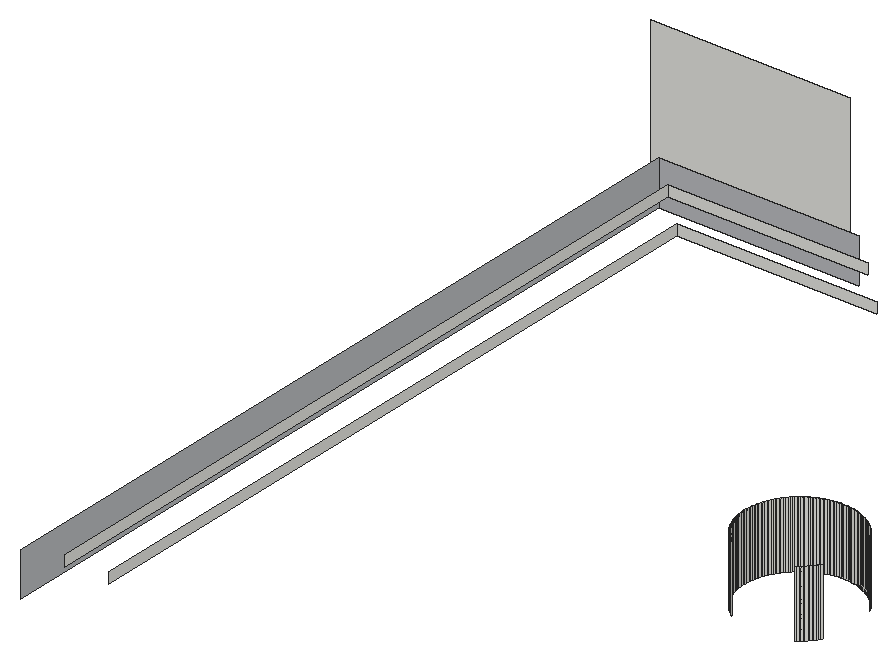
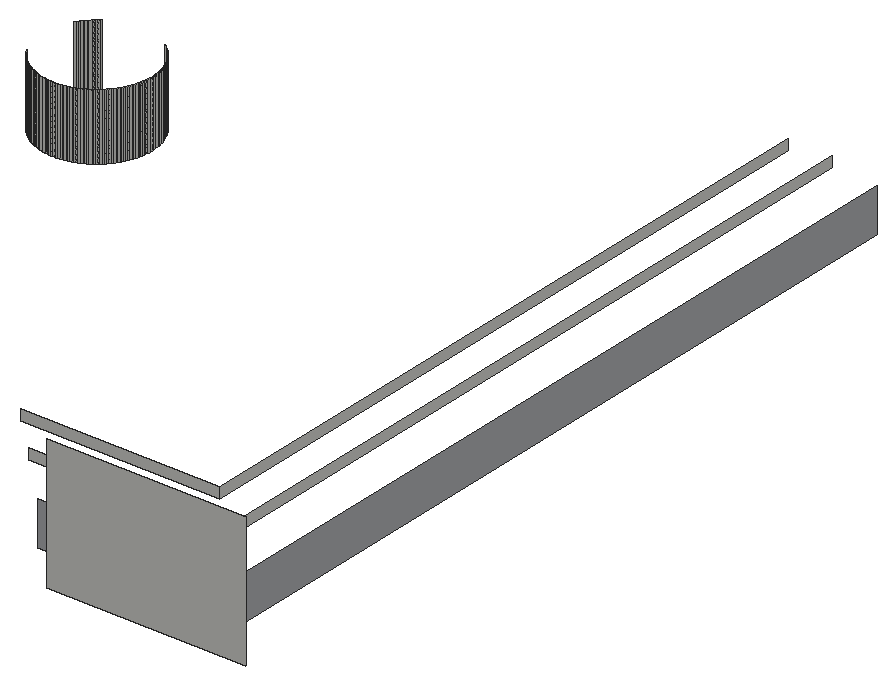
# SketchUp Ruby script. Lengths in inches.
U = 1.inch
M = Sketchup.active_model
def pt(a) = Geom::Point3d.new(a.map { |v| v * U })
def face(e, loops, mat)
  f = e.add_face(loops[0].map { |a| pt(a) })
  loops[1..].each { |l| e.add_face(l.map { |a| pt(a) }).erase! }
  f.material = f.back_material = mat if mat
  f
end
# faces: each face lists its corners as indices into pts; further lists are holes
def faces(e, pts, list, mat = nil) = list.each { |f| face(e, (f[0].is_a?(Array) ? f : [f]).map { |l| l.map { |i| pts[i] } }, mat) }
# xy, xz, yz: faces in a plane at the given z, y or x. An outline is a flat list of corners, or four numbers for a rectangle; further outlines are holes
def ring(l) = l.size == 4 ? [[l[0], l[1]], [l[2], l[1]], [l[2], l[3]], [l[0], l[3]]] : l.each_slice(2).to_a
def flat(e, list, mat, &to3) = list.each { |f| face(e, (f[0].is_a?(Array) ? f : [f]).map { |l| ring(l).map { |u, v| to3.(u, v) } }, mat) }
def xy(e, z, list, mat = nil) = flat(e, list, mat) { |x, y| [x, y, z] }
def xz(e, y, list, mat = nil) = flat(e, list, mat) { |x, z| [x, y, z] }
def yz(e, x, list, mat = nil) = flat(e, list, mat) { |y, z| [x, y, z] }
def lines(e, pts, list) = list.each { |a, b| e.add_line(pt(pts[a]), pt(pts[b])) }
# prism: a flat outline (further loops are holes) pulled along v
def prism(e, loops, v, mat = nil)
  f = face(e, loops, mat); d = Geom::Vector3d.new(v.map { |x| x * U })
  f.pushpull(f.normal.samedirection?(d) ? d.length : -d.length)
end
def box(e, o, s, mat = nil) = prism(e, [[o, [o[0] + s[0], o[1], o[2]], [o[0] + s[0], o[1] + s[1], o[2]], [o[0], o[1] + s[1], o[2]]]], [0, 0, s[2]], mat)
def at(x, y, z, deg = 0) = Geom::Transformation.translation(pt([x, y, z])) * Geom::Transformation.rotation(ORIGIN, Z_AXIS, deg.degrees)
def axes(o, x, y, z) = Geom::Transformation.new([*x, 0, *y, 0, *z, 0, *pt(o).to_a, 1])
def part(name) = M.definitions.add(name)
# library, detail: a bought-in or finely detailed component or shape, given as its bounding box
def library(name, o, s) = part(name).tap { |d| box(d.entities, o, s) }
def detail(e, o, s) = box(e.add_group.entities, o, s)
def put(e, d, t, mat = nil) = e.add_instance(d, t).tap { |i| i.material = mat if mat }
def group(e, t, mat = nil) = e.add_group.tap { |g| g.transformation = t; g.material = mat if mat }.entities
root = M.entities
M.materials.add("1427 AP 686 ARMOUR-N").color = [184, 186, 189]
xz(root,158.42,[[34.84,242,34.92,245],[34.92,242,35,245],[35,242,35.08,245],[35.08,242,35.16,245]])
xz(root,174,[[15,242,24,242.5]])
xz(root,176,[[13,242,22,242.5]])
xz(root,178,[[11,240,20,242]],"1427 AP 686 ARMOUR-N")
xz(root,180,[[9,240,18,246]])
yz(root,11,[[141.93,240,178,242]],"1427 AP 686 ARMOUR-N")
yz(root,13,[[141.9375,242,176,242.5]])
yz(root,15,[[141.94,242,174,242.5]])
yz(root,32.5,[[155.85,242,155.92,245],[155.92,242,156,245]])
yz(root,32.51,[[155.6875,242,155.77,245],[156.08,242,156.16,245]])
p = [[33.47,153.95,242],[33.41,154,242],[33.41,154,245],[33.47,153.95,245],[33.53,153.9,242],[33.53,153.9,245],
  [33.59,153.86,242],[33.59,153.86,245],[36.47,153.9,242],[36.41,153.86,242],[36.41,153.86,245],[36.47,153.9,245],
  [36.53,153.95,242],[36.53,153.95,245],[36.59,154,242],[36.59,154,245],[33.35,154.05,242],[33.29,154.1,242],
  [33.29,154.1,245],[33.35,154.05,245],[36.65,154.05,242],[36.65,154.05,245],[36.71,154.1,242],[36.71,154.1,245],
  [33.23,154.16,242],[33.23,154.16,245],[36.77,154.16,242],[36.77,154.16,245],[33.18,154.21,242],[33.125,154.27,242],
  [33.125,154.27,245],[33.18,154.21,245],[36.82,154.21,242],[36.82,154.21,245],[36.875,154.27,242],[36.875,154.27,245],
  [33.07,154.33,242],[33.02,154.39,242],[33.02,154.39,245],[33.07,154.33,245],[36.93,154.33,242],[36.93,154.33,245],
  [36.98,154.39,242],[36.98,154.39,245],[32.98,154.45,242],[32.98,154.45,245],[37.02,154.45,242],[37.02,154.45,245],
  [32.93,154.52,242],[32.89,154.58,242],[32.89,154.58,245],[32.93,154.52,245],[37.07,154.52,242],[37.07,154.52,245],
  [37.11,154.58,242],[37.11,154.58,245],[32.85,154.65,242],[32.85,154.65,245],[32.81,154.72,242],[32.77,154.79,242],
  [32.77,154.79,245],[32.81,154.72,245],[32.74,154.86,242],[32.74,154.86,245],[32.71,154.93,242],[32.68,155,242],
  [32.68,155,245],[32.71,154.93,245],[32.65,155.08,242],[32.65,155.08,245],[32.62,155.15,242],[32.62,155.15,245],
  [32.6,155.23,242],[32.58,155.3,242],[32.58,155.3,245],[32.6,155.23,245],[32.56,155.38,242],[32.56,155.38,245],
  [32.54,155.46,242],[32.54,155.46,245],[32.53,155.53,242],[32.52,155.61,242],[32.52,155.61,245],[32.53,155.53,245],
  [32.51,155.6875,242],[32.51,155.6875,245],[32.51,155.77,242],[32.5,155.85,242],[32.5,155.85,245],[32.51,155.77,245],
  [32.5,156,242],[32.51,156.08,242],[32.51,156.08,245],[32.5,156,245],[32.51,156.16,242],[32.52,156.24,242],
  [32.52,156.24,245],[32.51,156.16,245],[32.53,156.32,242],[32.53,156.32,245],[32.54,156.39,242],[32.54,156.39,245],
  [32.56,156.47,242],[32.56,156.47,245],[32.58,156.55,242],[32.58,156.55,245],[32.6,156.62,242],[32.6,156.62,245],
  [32.62,156.7,242],[32.62,156.7,245],[32.65,156.77,242],[32.65,156.77,245],[32.68,156.84,242],[32.68,156.84,245],
  [32.71,156.92,242],[32.71,156.92,245],[32.74,156.99,242],[32.74,156.99,245],[32.77,157.06,242],[32.77,157.06,245],
  [32.81,157.13,242],[32.81,157.13,245],[32.85,157.2,242],[32.85,157.2,245],[32.89,157.26,242],[32.89,157.26,245],
  [37.11,157.26,242],[37.15,157.2,242],[37.15,157.2,245],[37.11,157.26,245],[32.93,157.33,242],[32.93,157.33,245],
  [32.98,157.39,242],[32.98,157.39,245],[37.02,157.39,242],[37.07,157.33,242],[37.07,157.33,245],[37.02,157.39,245],
  [33.02,157.46,242],[33.02,157.46,245],[36.98,157.46,242],[36.98,157.46,245],[33.07,157.52,242],[33.07,157.52,245],
  [33.125,157.58,242],[33.125,157.58,245],[36.875,157.58,242],[36.93,157.52,242],[36.93,157.52,245],[36.875,157.58,245],
  [33.18,157.64,242],[33.18,157.64,245],[33.23,157.69,242],[33.23,157.69,245],[36.77,157.69,242],[36.82,157.64,242],
  [36.82,157.64,245],[36.77,157.69,245],[33.29,157.75,242],[33.29,157.75,245],[33.35,157.8,242],[33.35,157.8,245],
  [36.65,157.8,242],[36.71,157.75,242],[36.71,157.75,245],[36.65,157.8,245],[33.41,157.85,242],[33.41,157.85,245],
  [36.59,157.85,242],[36.59,157.85,245],[33.47,157.9,242],[33.47,157.9,245],[33.53,157.95,242],[33.53,157.95,245],
  [33.59,157.99,242],[33.59,157.99,245],[36.41,157.99,242],[36.47,157.95,242],[36.47,157.95,245],[36.41,157.99,245],
  [36.53,157.9,242],[36.53,157.9,245],[33.66,158.04,242],[33.66,158.04,245],[33.73,158.08,242],[33.73,158.08,245],
  [36.27,158.08,242],[36.34,158.04,242],[36.34,158.04,245],[36.27,158.08,245],[33.8,158.12,242],[33.8,158.12,245],
  [33.87,158.15,242],[33.87,158.15,245],[36.14,158.15,242],[36.2,158.12,242],[36.2,158.12,245],[36.14,158.15,245],
  [33.9375,158.1875,242],[33.9375,158.1875,245],[34.01,158.22,242],[34.01,158.22,245],[34.08,158.25,242],[34.08,158.25,245],
  [34.15,158.28,242],[34.15,158.28,245],[35.85,158.28,242],[35.92,158.25,242],[35.92,158.25,245],[35.85,158.28,245],
  [35.99,158.22,242],[35.99,158.22,245],[36.06,158.1875,242],[36.06,158.1875,245],[34.23,158.3,242],[34.23,158.3,245],
  [34.3,158.33,242],[34.3,158.33,245],[34.38,158.35,242],[34.38,158.35,245],[34.45,158.36,242],[34.45,158.36,245],
  [35.55,158.36,242],[35.62,158.35,242],[35.62,158.35,245],[35.55,158.36,245],[35.7,158.33,242],[35.7,158.33,245],
  [35.77,158.3,242],[35.77,158.3,245],[34.53,158.38,242],[34.53,158.38,245],[34.61,158.39,242],[34.61,158.39,245],
  [34.6875,158.4,242],[34.6875,158.4,245],[34.76,158.41,242],[34.76,158.41,245],[34.84,158.42,242],[34.84,158.42,245],
  [35.16,158.42,242],[35.24,158.41,242],[35.24,158.41,245],[35.16,158.42,245],[35.3125,158.4,242],[35.3125,158.4,245],
  [35.39,158.39,242],[35.39,158.39,245],[35.47,158.38,242],[35.47,158.38,245]]
faces(root,p,[[0,1,2,3],[4,0,3,5],[6,4,5,7],[8,9,10,11],[12,8,11,13],[14,12,13,15],[16,17,18,19],[1,16,19,2],
  [20,14,15,21],[22,20,21,23],[17,24,25,18],[26,22,23,27],[28,29,30,31],[24,28,31,25],[32,26,27,33],[34,32,33,35],
  [36,37,38,39],[29,36,39,30],[40,34,35,41],[42,40,41,43],[37,44,45,38],[46,42,43,47],[48,49,50,51],[44,48,51,45],
  [52,46,47,53],[54,52,53,55],[49,56,57,50],[58,59,60,61],[56,58,61,57],[59,62,63,60],[64,65,66,67],[62,64,67,63],
  [65,68,69,66],[68,70,71,69],[72,73,74,75],[70,72,75,71],[73,76,77,74],[76,78,79,77],[80,81,82,83],[78,80,83,79],
  [81,84,85,82],[86,87,88,89],[90,91,92,93],[94,95,96,97],[95,98,99,96],[98,100,101,99],[100,102,103,101],[102,104,105,103],
  [104,106,107,105],[106,108,109,107],[108,110,111,109],[110,112,113,111],[112,114,115,113],[114,116,117,115],[116,118,119,117],[118,120,121,119],
  [120,122,123,121],[122,124,125,123],[126,127,128,129],[124,130,131,125],[130,132,133,131],[134,135,136,137],[135,126,129,136],[132,138,139,133],
  [140,134,137,141],[138,142,143,139],[142,144,145,143],[146,147,148,149],[147,140,141,148],[144,150,151,145],[150,152,153,151],[154,155,156,157],
  [155,146,149,156],[152,158,159,153],[158,160,161,159],[162,163,164,165],[163,154,157,164],[160,166,167,161],[168,162,165,169],[166,170,171,167],
  [170,172,173,171],[172,174,175,173],[176,177,178,179],[177,180,181,178],[180,168,169,181],[174,182,183,175],[182,184,185,183],[186,187,188,189],
  [187,176,179,188],[184,190,191,185],[190,192,193,191],[194,195,196,197],[195,186,189,196],[192,198,199,193],[198,200,201,199],[200,202,203,201],
  [202,204,205,203],[206,207,208,209],[207,210,211,208],[210,212,213,211],[212,194,197,213],[204,214,215,205],[214,216,217,215],[216,218,219,217],
  [218,220,221,219],[222,223,224,225],[223,226,227,224],[226,228,229,227],[228,206,209,229],[220,230,231,221],[230,232,233,231],[232,234,235,233],
  [234,236,237,235],[236,238,239,237],[240,241,242,243],[241,244,245,242],[244,246,247,245],[246,248,249,247],[248,222,225,249]])
